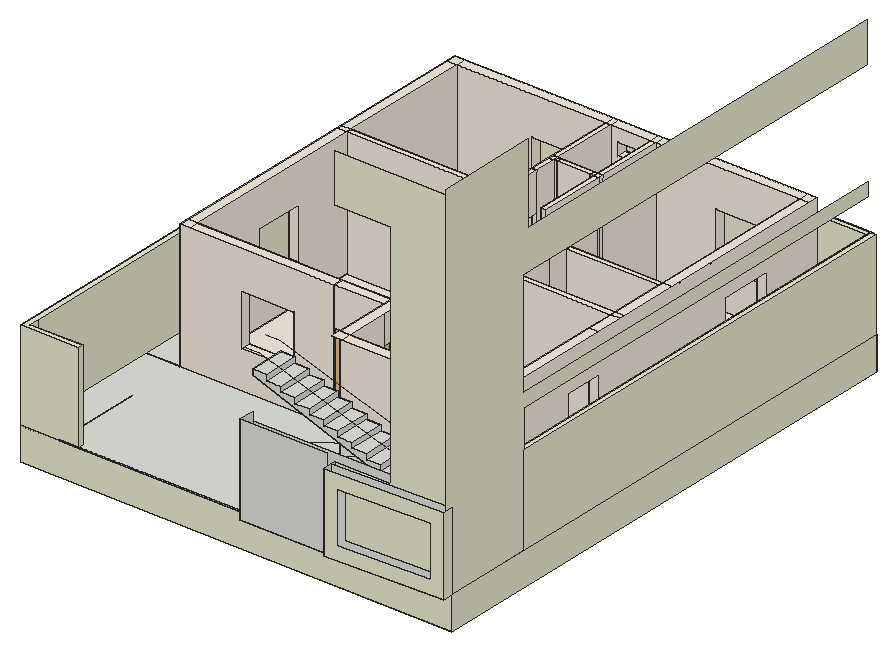
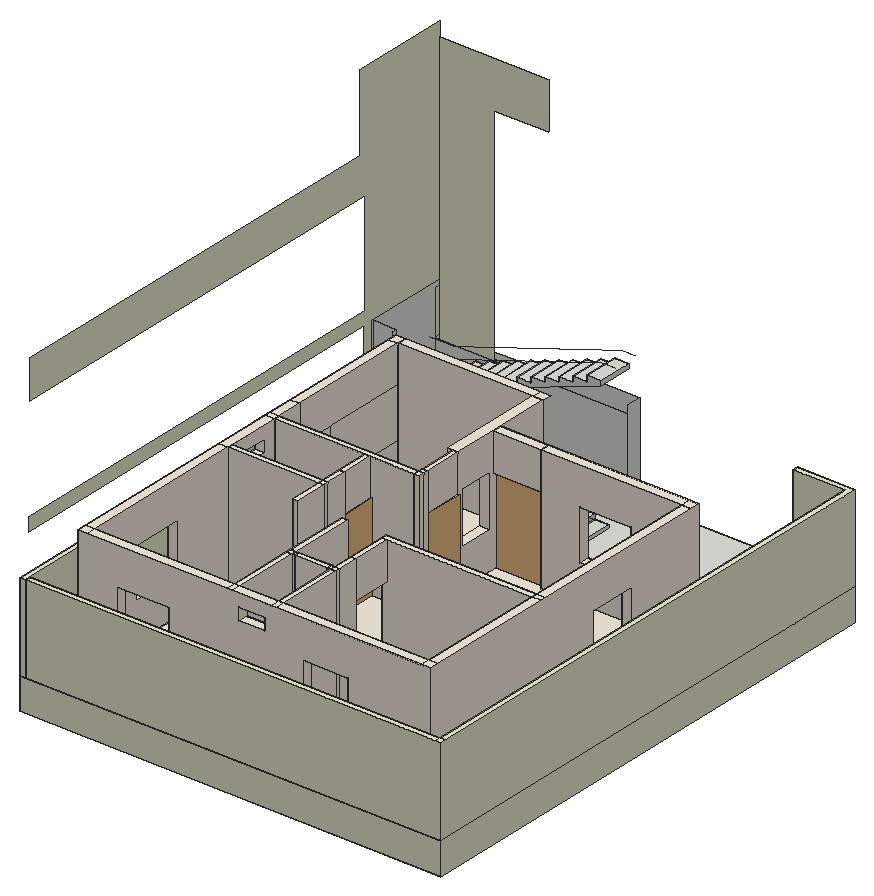
# SketchUp Ruby script. Lengths in inches.
U = 1.inch
M = Sketchup.active_model
def pt(a) = Geom::Point3d.new(a.map { |v| v * U })
def face(e, loops, mat)
  f = e.add_face(loops[0].map { |a| pt(a) })
  loops[1..].each { |l| e.add_face(l.map { |a| pt(a) }).erase! }
  f.material = f.back_material = mat if mat
  f
end
# faces: each face lists its corners as indices into pts; further lists are holes
def faces(e, pts, list, mat = nil) = list.each { |f| face(e, (f[0].is_a?(Array) ? f : [f]).map { |l| l.map { |i| pts[i] } }, mat) }
# xy, xz, yz: faces in a plane at the given z, y or x. An outline is a flat list of corners, or four numbers for a rectangle; further outlines are holes
def ring(l) = l.size == 4 ? [[l[0], l[1]], [l[2], l[1]], [l[2], l[3]], [l[0], l[3]]] : l.each_slice(2).to_a
def flat(e, list, mat, &to3) = list.each { |f| face(e, (f[0].is_a?(Array) ? f : [f]).map { |l| ring(l).map { |u, v| to3.(u, v) } }, mat) }
def xy(e, z, list, mat = nil) = flat(e, list, mat) { |x, y| [x, y, z] }
def xz(e, y, list, mat = nil) = flat(e, list, mat) { |x, z| [x, y, z] }
def yz(e, x, list, mat = nil) = flat(e, list, mat) { |y, z| [x, y, z] }
def lines(e, pts, list) = list.each { |a, b| e.add_line(pt(pts[a]), pt(pts[b])) }
# prism: a flat outline (further loops are holes) pulled along v
def prism(e, loops, v, mat = nil)
  f = face(e, loops, mat); d = Geom::Vector3d.new(v.map { |x| x * U })
  f.pushpull(f.normal.samedirection?(d) ? d.length : -d.length)
end
def box(e, o, s, mat = nil) = prism(e, [[o, [o[0] + s[0], o[1], o[2]], [o[0] + s[0], o[1] + s[1], o[2]], [o[0], o[1] + s[1], o[2]]]], [0, 0, s[2]], mat)
def at(x, y, z, deg = 0) = Geom::Transformation.translation(pt([x, y, z])) * Geom::Transformation.rotation(ORIGIN, Z_AXIS, deg.degrees)
def axes(o, x, y, z) = Geom::Transformation.new([*x, 0, *y, 0, *z, 0, *pt(o).to_a, 1])
def part(name) = M.definitions.add(name)
# library, detail: a bought-in or finely detailed component or shape, given as its bounding box
def library(name, o, s) = part(name).tap { |d| box(d.entities, o, s) }
def detail(e, o, s) = box(e.add_group.entities, o, s)
def put(e, d, t, mat = nil) = e.add_instance(d, t).tap { |i| i.material = mat if mat }
def group(e, t, mat = nil) = e.add_group.tap { |g| g.transformation = t; g.material = mat if mat }.entities
root = M.entities
M.materials.add("0037 AP 8028 PEACH ORGANZA").color = [246, 236, 223]
M.materials.add("0746 AP 7715 LUMINOUS").color = [235, 235, 209]
c1 = library("Group\#12",[0,0,0],[6.9375,42,86.5])
c2 = part("Group19\#2")
p = [[1706.5625,247.76,0],[1706.5625,271.76,0],[1706.5625,427.76,65],[1706.5625,431.76,65],[1720.5625,431.76,65],[1720.5625,427.76,65],
  [1720.5625,283.76,125],[1720.5625,271.76,125],[1686.5625,247.76,0],[1686.5625,271.76,0],[1686.5625,427.76,65],[1686.5625,451.76,65],
  [1740.5625,451.76,65],[1740.5625,427.76,65],[1740.5625,283.76,125],[1740.5625,271.76,125]]
lines(c2.entities,p,[[0,1],[1,2],[2,3],[3,4],[4,5],[5,6],[6,7],[8,9],[9,10],[10,11],[11,12],[12,13],
  [13,14],[14,15]])
c3 = part("Group18\#1")
xy(c3.entities,-3.9375,[[1682.5625,269.14,1710.5625,281.14],[1682.5625,281.14,1710.5625,281.93]])
xy(c3.entities,0.45,[[1682.5625,269.14,1710.5625,281.14]])
xy(c3.entities,6.01,[[1682.5625,281.14,1710.5625,293.14]])
xy(c3.entities,11.58,[[1682.5625,293.14,1710.5625,305.14]])
xy(c3.entities,17.14,[[1682.5625,305.14,1710.5625,317.14]])
xy(c3.entities,22.71,[[1682.5625,317.14,1710.5625,329.14]])
xy(c3.entities,28.27,[[1682.5625,329.14,1710.5625,341.14]])
xy(c3.entities,33.84,[[1682.5625,341.14,1710.5625,353.14]])
xy(c3.entities,39.4,[[1682.5625,353.14,1710.5625,365.14]])
xy(c3.entities,44.97,[[1682.5625,365.14,1710.5625,377.14]])
xy(c3.entities,50.53,[[1682.5625,377.14,1710.5625,389.14]])
xy(c3.entities,56.1,[[1682.5625,389.14,1710.5625,401.14]])
xy(c3.entities,61.66,[[1682.5625,401.14,1710.5625,413.14]])
xy(c3.entities,67.23,[[1682.5625,413.14,1710.5625,425.14]])
xy(c3.entities,68.41,[[1716.5625,412.36,1744.5625,453.14],[1710.5625,425.14,1710.5625,437.93,1682.5625,437.93,1682.5625,453.14,1716.5625,453.14,1716.5625,425.14]])
xy(c3.entities,72.8,[[1716.5625,413.14,1744.5625,453.14],[1682.5625,425.14,1716.5625,453.14]])
xy(c3.entities,78.36,[[1716.5625,401.14,1744.5625,413.14]])
xy(c3.entities,83.93,[[1716.5625,389.14,1744.5625,401.14]])
xy(c3.entities,89.49,[[1716.5625,377.14,1744.5625,389.14]])
xy(c3.entities,95.06,[[1716.5625,365.14,1744.5625,377.14]])
xy(c3.entities,100.62,[[1716.5625,353.14,1744.5625,365.14]])
xy(c3.entities,106.1875,[[1716.5625,341.14,1744.5625,353.14]])
xy(c3.entities,111.75,[[1716.5625,329.14,1744.5625,341.14]])
xy(c3.entities,117.32,[[1716.5625,317.14,1744.5625,329.14]])
xy(c3.entities,122.88,[[1716.5625,305.14,1744.5625,317.14]])
xy(c3.entities,128.45,[[1716.5625,293.14,1744.5625,305.14]])
xy(c3.entities,134.68,[[1716.5625,281.14,1744.5625,293.14]])
xz(c3.entities,269.14,[[1682.5625,-3.9375,1710.5625,0.45]])
xz(c3.entities,281.14,[[1682.5625,-3.9375,1710.5625,0.45],[1682.5625,0.45,1710.5625,6.01],[1716.5625,129.27,1744.5625,134.68]])
xz(c3.entities,293.14,[[1682.5625,6.01,1710.5625,11.58],[1716.5625,128.45,1744.5625,134.68]])
xz(c3.entities,305.14,[[1682.5625,11.58,1710.5625,17.14],[1716.5625,122.88,1744.5625,128.45]])
xz(c3.entities,317.14,[[1682.5625,17.14,1710.5625,22.71],[1716.5625,117.32,1744.5625,122.88]])
xz(c3.entities,329.14,[[1682.5625,22.71,1710.5625,28.27],[1716.5625,111.75,1744.5625,117.32]])
xz(c3.entities,341.14,[[1682.5625,28.27,1710.5625,33.84],[1716.5625,106.1875,1744.5625,111.75]])
xz(c3.entities,353.14,[[1682.5625,33.84,1710.5625,39.4],[1716.5625,100.62,1744.5625,106.1875]])
xz(c3.entities,365.14,[[1682.5625,39.4,1710.5625,44.97],[1716.5625,95.06,1744.5625,100.62]])
xz(c3.entities,377.14,[[1682.5625,44.97,1710.5625,50.53],[1716.5625,89.49,1744.5625,95.06]])
xz(c3.entities,389.14,[[1682.5625,50.53,1710.5625,56.1],[1716.5625,83.93,1744.5625,89.49]])
xz(c3.entities,401.14,[[1682.5625,56.1,1710.5625,61.66],[1716.5625,78.36,1744.5625,83.93]])
xz(c3.entities,413.14,[[1682.5625,61.66,1710.5625,67.23],[1716.5625,72.8,1744.5625,78.36]])
xz(c3.entities,425.14,[[1682.5625,67.23,1710.5625,72.8],[1710.5625,68.41,1716.5625,72.8]])
xz(c3.entities,453.14,[[1682.5625,68.41,1716.5625,72.8],[1716.5625,68.41,1744.5625,72.8]])
yz(c3.entities,1682.5625,[[269.14,-3.9375,281.14,0.45],[281.14,-3.9375,281.14,6.01,293.14,6.01,293.14,11.58,305.14,11.58,305.14,17.14,317.14,17.14,317.14,22.71,329.14,22.71,329.14,28.27,341.14,28.27,341.14,33.84,353.14,33.84,353.14,39.4,365.14,39.4,365.14,44.97,377.14,44.97,377.14,50.53,389.14,50.53,389.14,56.1,401.14,56.1,401.14,61.66,413.14,61.66,413.14,67.23,425.14,67.23,425.14,72.8,453.14,72.8,453.14,68.41,437.93,68.41,281.93,-3.9375]])
yz(c3.entities,1710.5625,[[269.14,-3.9375,281.14,0.45],[281.14,-3.9375,281.93,-3.9375,437.93,68.41,425.14,68.41,425.14,67.23,413.14,67.23,413.14,61.66,401.14,61.66,401.14,56.1,389.14,56.1,389.14,50.53,377.14,50.53,377.14,44.97,365.14,44.97,365.14,39.4,353.14,39.4,353.14,33.84,341.14,33.84,341.14,28.27,329.14,28.27,329.14,22.71,317.14,22.71,317.14,17.14,305.14,17.14,305.14,11.58,293.14,11.58,293.14,6.01,281.14,6.01]])
yz(c3.entities,1716.5625,[[412.36,68.41,281.42,129.14,281.14,129.27,281.14,134.68,293.14,134.68,293.14,128.45,305.14,128.45,305.14,122.88,317.14,122.88,317.14,117.32,329.14,117.32,329.14,111.75,341.14,111.75,341.14,106.1875,353.14,106.1875,353.14,100.62,365.14,100.62,365.14,95.06,377.14,95.06,377.14,89.49,389.14,89.49,389.14,83.93,401.14,83.93,401.14,78.36,413.14,78.36,413.14,72.8,425.14,72.8,425.14,68.41],[425.14,68.41,453.14,72.8]])
yz(c3.entities,1744.5625,[[412.36,68.41,453.14,68.41,453.14,72.8,413.14,72.8,413.14,78.36,401.14,78.36,401.14,83.93,389.14,83.93,389.14,89.49,377.14,89.49,377.14,95.06,365.14,95.06,365.14,100.62,353.14,100.62,353.14,106.1875,341.14,106.1875,341.14,111.75,329.14,111.75,329.14,117.32,317.14,117.32,317.14,122.88,305.14,122.88,305.14,128.45,293.14,128.45,293.14,134.68,281.14,134.68,281.14,129.27]])
p = [[1682.5625,281.93,-3.9375],[1682.5625,437.93,68.41],[1710.5625,437.93,68.41],[1710.5625,281.93,-3.9375],[1744.5625,412.36,68.41],[1744.5625,281.14,129.27],
  [1716.5625,281.42,129.14],[1716.5625,412.36,68.41],[1716.5625,281.14,129.27]]
faces(c3.entities,p,[[0,1,2,3],[4,5,6,7],[8,6,5]])
put(c3.entities,c2,at(0,0,24))
xy(root,-0.68,[[2448.97,99.37,2448.64,108.36,2554.91,112.36,2555.24,103.37],[2370.2,103.36,2370.2,112.52,2550.375,112.52,2550.375,112.36,2448.64,112.36,2448.64,103.36],[2448.64,108.36,2448.64,112.36,2554.91,112.36],[2550.375,112.36,2554.91,112.52],[2370.2,112.52,2550.375,117.53],
  [2550.375,112.52,2554.91,191.07],[2550.375,191.07,2554.91,194.04],[2463.86,337.26,2499.86,337.34,2499.86,337.47,2463.86,337.39]])
xz(root,103.36,[[2370.2,-0.68,2448.64,-0.68,2448.64,69.55,2448.6,69.55,2448.6,80.8,2370.2,80.8]])
xz(root,112.36,[[2448.64,-0.68,2554.91,-0.68,2554.91,69.55,2549.9,69.55,2549.9,322.5,2448.6,322.5,2448.6,278.5,2499.54,278.5,2499.54,69.55,2448.64,69.55]],"0746 AP 7715 LUMINOUS")
xz(root,117.53,[[2370.2,-0.68,2370.2,73.55,2549.9,73.55,2549.9,115.5,2550.375,115.5,2550.375,-0.68]])
xz(root,190.04,[[2528.375,-0.68,2550.375,120]])
yz(root,2370.2,[[103.36,-0.68,103.36,80.8,117.37,80.8,117.37,73.55,117.53,73.55,117.53,-0.68]])
yz(root,2448.64,[[103.36,-0.68,108.36,69.55],[108.36,-0.68,112.36,69.55]])
yz(root,2528.375,[[190.04,-0.68,194.04,120]])
yz(root,2550.375,[[117.53,-0.68,117.53,115.5,112.36,115.5,112.36,120,190.04,120,190.04,-0.68],[190.04,-0.68,191.07,120]])
yz(root,2554.91,[[112.36,-0.68,194.04,-0.68,194.04,115.5,584.4,115.5,584.4,127.5,192.78,127.5,192.78,223.5,583.09,223.5,583.09,259.5,198.89,259.5,198.89,331.5,105.36,331.5,105.36,69.55,112.36,69.55]],"0746 AP 7715 LUMINOUS")
p = [[2448.64,108.36,69.55],[2448.64,108.36,-0.68],[2448.97,99.37,-0.68],[2448.97,99.37,69.55],[2555.24,103.37,69.55],[2555.24,103.37,-0.68],
  [2543.25,102.92,11.32],[2460.97,99.82,11.32],[2460.97,99.82,57.55],[2543.25,102.92,57.55],[2554.91,112.36,-0.68],[2554.91,112.36,69.55],
  [2499.54,110.28,69.55],[2549.9,112.18,69.55],[2460.625,108.82,11.32],[2542.91,111.91,11.32],[2542.91,111.91,57.55],[2499.54,110.28,57.55],
  [2460.625,108.82,57.55]]
faces(root,p,[[0,1,2,3],[[0,12,13,11,10,1],[14,15,16,17,18]]])
faces(root,p,[[[4,3,2,5],[6,7,8,9]],[10,11,4,5]],"0746 AP 7715 LUMINOUS")
g1 = group(root,at(2163.39,579.02,-0.68),"0746 AP 7715 LUMINOUS")
xy(g1,0,[[0,-466.5,5.01,-461.49],[5.01,-466.5,53.01,-461.49],[0,-461.49,5.01,-452.29],[0,-452.29,5.01,9.73],[386.98,-384.97,391.99,14.74],
  [0,9.73,5.01,14.74],[5.01,9.73,386.98,14.74]])
xy(g1,81.48,[[0,-466.5,53.01,-466.5,53.01,-461.49,5.01,-461.49,5.01,9.73,0,9.73],[386.98,-384.97,391.99,14.74],[0,9.73,5.01,14.74],[5.01,9.73,386.98,14.74]])
xz(g1,-466.5,[[0,0,53.01,81.48]])
xz(g1,-461.49,[[5.01,0,53.01,81.48]])
xz(g1,-384.97,[[386.98,0,391.99,81.48]])
xz(g1,9.73,[[5.01,0,386.98,81.48]])
xz(g1,14.74,[[0,0,386.98,81.48],[386.98,0,391.99,81.48]])
yz(g1,0,[[-466.5,0,14.74,81.48]])
yz(g1,5.01,[[-461.49,0,-452.29,81.48],[-452.29,0,9.73,81.48]])
yz(g1,53.01,[[-466.5,0,-461.49,81.48]])
yz(g1,386.98,[[-384.97,0,9.73,81.48],[9.73,0,14.74,81.48]])
yz(g1,391.99,[[-384.97,0,14.74,81.48]])
g2 = group(root,at(2168.4,553.29,-0.68))
xy(g2,0,[[-5.01,-440.77,-5.01,40.47,386.98,40.47,386.98,-440.77,381.97,-440.77,381.97,35.34,0,35.34,0,-435.76,30.99,-435.76,30.99,-440.77],[30.99,-440.77,381.97,-359.24],[0,-435.76,0,-304.77,215.96,-304.77,215.96,-359.24,30.99,-359.24,30.99,-435.76],[359.97,-359.24,381.97,7.26],[0,-304.77,30.99,0],
  [0,0,30.99,7.26],[0,7.26,30.99,35.34],[30.99,7.26,359.97,35.34],[359.97,7.26,381.97,35.34]])
xy(g2,0.97,[[30.99,-440.77,381.97,-440.77,381.97,-359.24,215.96,-359.24,215.96,-304.77,0,-304.77,0,-435.76,30.99,-435.76],[359.97,-359.24,381.97,7.26],[0,-304.77,30.99,0],[0,0,30.99,7.26],[0,7.26,30.99,35.34],
  [30.99,7.26,359.97,35.34],[359.97,7.26,381.97,35.34]])
xz(g2,-440.77,[[30.99,0,381.97,0.97]])
xz(g2,-435.76,[[0,0,30.99,0.97]])
xz(g2,-359.24,[[215.96,0,359.97,0.97]])
xz(g2,-304.77,[[0,0,30.99,0.97],[30.99,0,215.96,0.97]])
xz(g2,0,[[0,0,30.99,0.97]])
xz(g2,7.26,[[0,0,30.99,0.97],[30.99,0,359.97,0.97],[359.97,0,381.97,0.97]])
xz(g2,35.34,[[0,0,30.99,0.97],[30.99,0,359.97,0.97],[359.97,0,381.97,0.97]])
yz(g2,0,[[-435.76,0,-304.77,0.97],[-304.77,0,0,0.97],[0,0,7.26,0.97],[7.26,0,35.34,0.97]])
yz(g2,30.99,[[-440.77,0,-435.76,0.97],[-435.76,0,-359.24,0.97],[-304.77,0,0,0.97],[0,0,7.26,0.97],[7.26,0,35.34,0.97]])
yz(g2,215.96,[[-359.24,0,-304.77,0.97]])
yz(g2,359.97,[[-359.24,0,7.26,0.97],[7.26,0,35.34,0.97]])
yz(g2,381.97,[[-440.77,0,-359.24,0.97],[-359.24,0,7.26,0.97],[7.26,0,35.34,0.97]])
g3 = group(root,at(2163.39,112.52,-30.68),"0746 AP 7715 LUMINOUS")
box(g3,[0,0,0],[392,481.24,30])
put(root,c1,axes([2384.37,249.12,-0.68],[0,0.7279,0],[-1.06713,0,0],[0,0,0.94197]))
g4 = group(root,at(2199.39,551.55,-0.68),"0037 AP 8028 PEACH ORGANZA")
xy(g4,0,[[184.97,-361.51,194,-352.52],[194,-361.51,319.99,-352.52],[319.99,-361.51,328.98,-352.52],[184.97,-352.52,194,-303.04],[194,-352.52,319.99,-303.04],
  [319.99,-352.52,328.98,-303.04],[0,-303.04,8.99,-294.03],[8.99,-303.04,140.15,-294.03],[184.97,-303.04,194,-253.68],[319.99,-303.04,328.98,-238.48],
  [0,-294.03,8.99,-294],[0,-294,8.99,-125],[319.99,-238.48,328.98,-214.09],[184.97,-218.02,189.98,-214.09],[184.97,-214.09,189.98,-209.03],
  [189.98,-214.09,319.99,-209.03],[319.99,-214.09,328.98,-209.03],[319.99,-209.03,328.98,-155.01],[230.99,-179.02,236,-160.01],[230.99,-160.01,236,-155.01],
  [236,-160.01,319.99,-155.01],[230.99,-155.01,236,-125],[319.99,-155.01,328.98,0],[0,-125,8.99,-120.03],[8.99,-125,148.97,-120.03],
  [184.97,-125,189.98,-65.02],[0,-120.03,8.99,0],[144,-84.03,148.97,-65.02],[144,-65.02,148.97,-60.02],[148.97,-65.02,151.97,-60.02],
  [181.98,-65.02,184.97,-60.02],[184.97,-65.02,189.98,-60.02],[144,-60.02,148.97,0],[184.97,-60.02,189.98,0],[0,0,8.99,8.99],
  [8.99,0,144,8.99],[144,0,148.97,8.99],[148.97,0,184.97,8.99],[184.97,0,189.98,8.99],[189.98,0,319.99,8.99],
  [319.99,0,328.98,8.99]])
xy(g4,34.92,[[319.99,-352.52,328.98,-274.28],[55.86,-303.04,103.86,-294.03],[319.99,-274.28,328.98,-238.48],[0,-225,8.99,-179.55],[319.99,-96,328.98,-48],
  [77.49,0,118.65,8.99],[244.5,0,291.95,8.99]])
xy(g4,35.49,[[184.97,-290.84,194,-258.52]])
xy(g4,81.32,[[0,-225,8.99,-179.55]])
xy(g4,81.38,[[77.49,0,118.65,8.99]])
xy(g4,81.48,[[55.86,-303.04,103.86,-294.03],[140.15,-303.04,184.97,-294.03],[319.99,-274.28,328.98,-238.48],[184.97,-253.68,189.49,-218.02],[230.99,-209.03,236.12,-179.02],
  [144,-120.03,148.97,-84.03],[319.99,-96,328.98,-48],[151.97,-65.02,181.98,-60.02],[244.5,0,291.95,8.99]])
xy(g4,83.3,[[184.97,-290.84,194,-258.52]])
xy(g4,93.12,[[319.99,-197.03,328.98,-172.01],[154.97,0,178.97,8.99]])
xy(g4,104.76,[[319.99,-197.03,328.98,-172.01],[154.97,0,178.97,8.99]])
xy(g4,116.4,[[184.97,-361.51,194,-352.52],[194,-361.51,319.99,-352.52],[319.99,-361.51,328.98,-352.52],[184.97,-352.52,194,-253.68],[319.99,-352.52,328.98,-238.48],
  [0,-303.04,8.99,-294.03],[8.99,-303.04,140.15,-294.03],[140.15,-303.04,184.97,-294.03],[0,-294.03,8.99,-294],[0,-294,8.99,-125],
  [184.97,-253.68,189.49,-218.02],[319.99,-238.48,328.98,-214.09],[184.97,-218.02,189.98,-214.09],[184.97,-214.09,189.98,-209.03],[189.98,-214.09,319.99,-209.03],
  [319.99,-214.09,328.98,-209.03],[230.99,-209.03,236.12,-179.02],[319.99,-209.03,328.98,-155.01],[230.99,-179.02,236,-160.01],[230.99,-160.01,236,-155.01],
  [236,-160.01,319.99,-155.01],[230.99,-155.01,236,-125],[319.99,-155.01,328.98,0],[0,-125,8.99,-120.03],[8.99,-125,148.97,-120.03],
  [184.97,-125,189.98,-65.02],[0,-120.03,8.99,0],[144,-120.03,148.97,-84.03],[144,-84.03,148.97,-65.02],[144,-65.02,148.97,-60.02],
  [148.97,-65.02,151.97,-60.02],[151.97,-65.02,181.98,-60.02],[181.98,-65.02,184.97,-60.02],[184.97,-65.02,189.98,-60.02],[144,-60.02,148.97,0],
  [184.97,-60.02,189.98,0],[0,0,8.99,8.99],[8.99,0,144,8.99],[144,0,148.97,8.99],[148.97,0,184.97,8.99],
  [184.97,0,189.98,8.99],[189.98,0,319.99,8.99],[319.99,0,328.98,8.99]])
xz(g4,-361.51,[[319.99,0,328.98,116.4]])
xz(g4,-352.52,[[184.97,0,319.99,116.4],[319.99,0,328.98,34.92]])
xz(g4,-303.04,[[[0,0,140.15,116.4],[55.86,34.92,103.86,81.48]],[140.15,81.48,184.97,116.4]],"0037 AP 8028 PEACH ORGANZA")
xz(g4,-294.03,[[[8.99,0,140.15,116.4],[55.86,34.92,103.86,81.48]],[140.15,81.48,184.97,116.4]])
xz(g4,-290.84,[[184.97,35.49,194,83.3]])
xz(g4,-274.28,[[319.99,34.92,328.98,81.48]])
xz(g4,-258.52,[[184.97,35.49,194,83.3]])
xz(g4,-253.68,[[184.97,0,184.97,81.48,189.49,81.48,189.49,116.4,194,116.4,194,0],[184.97,81.48,189.49,116.4]])
xz(g4,-238.48,[[319.99,0,328.98,34.92],[319.99,34.92,328.98,81.48]])
xz(g4,-225,[[0,34.92,8.99,81.32]])
xz(g4,-218.02,[[184.97,0,189.98,0,189.98,116.4,189.49,116.4,189.49,81.48,184.97,81.48],[184.97,81.48,189.49,116.4]])
xz(g4,-214.09,[[184.97,0,189.98,116.4],[189.98,0,319.99,116.4]])
xz(g4,-209.03,[[184.97,0,189.98,116.4],[189.98,0,189.98,116.4,230.99,116.4,230.99,81.48,236.12,81.48,236.12,116.4,319.99,116.4,319.99,0],[230.99,81.48,236.12,116.4]])
xz(g4,-197.03,[[319.99,93.12,328.98,104.76]])
xz(g4,-179.55,[[0,34.92,8.99,81.32]])
xz(g4,-179.02,[[230.99,0,236,81.48],[230.99,81.48,236,116.4],[236,81.48,236.12,116.4]])
xz(g4,-172.01,[[319.99,93.12,328.98,104.76]])
xz(g4,-160.01,[[230.99,0,236,116.4],[236,0,319.99,116.4]])
xz(g4,-155.01,[[230.99,0,236,116.4],[236,0,319.99,116.4]])
xz(g4,-125,[[8.99,0,148.97,116.4],[184.97,0,189.98,116.4],[230.99,0,236,116.4]])
xz(g4,-120.03,[[8.99,0,8.99,116.4,144,116.4,144,81.48,148.97,81.48,148.97,0],[144,81.48,148.97,116.4]])
xz(g4,-96,[[319.99,34.92,328.98,81.48]])
xz(g4,-84.03,[[144,0,148.97,81.48],[144,81.48,148.97,116.4]])
xz(g4,-65.02,[[144,0,148.97,116.4],[148.97,0,151.97,116.4],[181.98,0,184.97,116.4],[184.97,0,189.98,116.4],[151.97,81.48,181.98,116.4]])
xz(g4,-60.02,[[144,0,148.97,116.4],[148.97,0,151.97,116.4],[181.98,0,184.97,116.4],[184.97,0,189.98,116.4],[151.97,81.48,181.98,116.4]])
xz(g4,-48,[[319.99,34.92,328.98,81.48]])
xz(g4,0,[[[8.99,0,144,116.4],[77.49,34.92,118.65,81.38]],[144,0,148.97,116.4],[[148.97,0,184.97,116.4],[154.97,93.12,178.97,104.76]],[184.97,0,189.98,116.4],[[189.98,0,319.99,116.4],[244.5,34.92,291.95,81.48]]])
xz(g4,8.99,[[[0,0,328.98,116.4],[244.5,34.92,291.95,81.48],[77.49,34.92,118.65,81.38],[154.97,93.12,178.97,104.76]]])
yz(g4,0,[[[-303.04,0,8.99,116.4],[-225,34.92,-179.55,81.32]]],"0037 AP 8028 PEACH ORGANZA")
yz(g4,8.99,[[-294.03,0,-294,116.4],[[-294,0,-125,116.4],[-225,34.92,-179.55,81.32]],[-125,0,-120.03,116.4],[-120.03,0,0,116.4]])
yz(g4,55.86,[[-303.04,34.92,-294.03,81.48]])
yz(g4,77.49,[[0,34.92,8.99,81.38]])
yz(g4,103.86,[[-303.04,34.92,-294.03,81.48]])
yz(g4,118.65,[[0,34.92,8.99,81.38]])
yz(g4,140.15,[[-303.04,0,-294.03,81.48],[-303.04,81.48,-294.03,116.4]])
yz(g4,144,[[-84.03,0,-65.02,116.4],[-65.02,0,-60.02,116.4],[-60.02,0,0,116.4],[-120.03,81.48,-84.03,116.4]])
yz(g4,148.97,[[-125,0,-120.03,116.4],[-84.03,0,-65.02,116.4],[-65.02,0,-60.02,116.4],[-60.02,0,0,116.4],[-120.03,81.48,-84.03,116.4]])
yz(g4,151.97,[[-65.02,0,-60.02,81.48],[-65.02,81.48,-60.02,116.4]])
yz(g4,154.97,[[0,93.12,8.99,104.76]])
yz(g4,178.97,[[0,93.12,8.99,104.76]])
yz(g4,181.98,[[-65.02,0,-60.02,81.48],[-65.02,81.48,-60.02,116.4]])
yz(g4,184.97,[[[-352.52,0,-352.52,116.4,-303.04,116.4,-303.04,81.48,-294.03,81.48,-294.03,116.4,-253.68,116.4,-253.68,0],[-290.84,35.49,-258.52,83.3]],[-218.02,0,-214.09,116.4],[-214.09,0,-209.03,116.4],[-125,0,-65.02,116.4],[-65.02,0,-60.02,116.4],
  [-60.02,0,0,116.4],[-303.04,81.48,-294.03,116.4],[-253.68,81.48,-218.02,116.4]])
yz(g4,189.49,[[-253.68,81.48,-218.02,116.4]])
yz(g4,189.98,[[-218.02,0,-214.09,116.4],[-214.09,0,-209.03,116.4],[-125,0,-65.02,116.4],[-65.02,0,-60.02,116.4],[-60.02,0,0,116.4]])
yz(g4,230.99,[[-179.02,0,-160.01,116.4],[-160.01,0,-155.01,116.4],[-155.01,0,-125,116.4],[-209.03,81.48,-179.02,116.4]])
yz(g4,236,[[-179.02,0,-160.01,116.4],[-160.01,0,-155.01,116.4],[-155.01,0,-125,116.4]])
yz(g4,236.12,[[-209.03,81.48,-179.02,116.4]])
yz(g4,244.5,[[0,34.92,8.99,81.48]])
yz(g4,291.95,[[0,34.92,8.99,81.48]])
yz(g4,319.99,[[-361.51,0,-352.52,116.4],[-352.52,0,-280.02,34.92],[-280.02,0,-238.48,34.92],[-238.48,0,-214.09,116.4],[-214.09,0,-209.03,116.4],
  [[-209.03,0,-160.01,116.4],[-197.03,93.12,-172.01,104.76]],[-160.01,0,-155.01,116.4],[[-155.01,0,0,116.4],[-96,34.92,-48,81.48]],[-352.52,34.92,-274.28,81.48],[-352.52,81.48,-238.48,116.4]])
yz(g4,328.98,[[[-361.51,0,-352.52,0,-352.52,34.92,-274.28,34.92,-274.28,81.48,-238.48,81.48,-238.48,0,8.99,0,8.99,116.4,-361.51,116.4],[-96,34.92,-48,81.48],[-197.03,93.12,-172.01,104.76]],[-352.52,0,-238.48,34.92]])
# 3 loose lines left out
g5 = group(g4,at(8.99,-303.04,0))
prism(g5,[[[311,0,0],[185.01,0,0],[185.01,49.36,0],[175.98,49.36,0],[175.98,0,0],[131.16,0,0],[131.16,9.01,0],[0,9.01,0],[0,9.03,0],[0,178.04,0],[139.98,178.04,0],[139.98,183,0],[0,183,0],[0,303.04,0],[135.02,303.04,0],[135.02,243.02,0],[135.02,238.01,0],[135.02,219,0],[139.98,219,0],[139.98,238.01,0],[142.98,238.01,0],[142.98,243.02,0],[139.98,243.02,0],[139.98,303.04,0],[175.98,303.04,0],[175.98,243.02,0],[172.99,243.02,0],[172.99,238.01,0],[175.98,238.01,0],[175.98,178.04,0],[180.99,178.04,0],[180.99,238.01,0],[180.99,243.02,0],[180.99,303.04,0],[311,303.04,0],[311,148.03,0],[227.01,148.03,0],[227.01,178.04,0],[222,178.04,0],[222,148.03,0],[222,143.02,0],[222,124.01,0],[227.01,124.01,0],[227.01,143.02,0],[311,143.02,0],[311,94.01,0],[180.99,94.01,0],[175.98,94.01,0],[175.98,88.95,0],[175.98,85.02,0],[180.99,85.02,0],[180.99,88.95,0],[311,88.95,0],[311,64.55,0],[311,23.02,0]]],[0,0,0.97])
put(root,c1,axes([2382.07,486.49,-0.68],[0,0.7279,0],[-0.73015,0,0],[0,0,0.94197]))
put(root,c1,axes([2382.94,297.875,-0.68],[0.85622,0,0],[0,0.84902,0],[0,0,0.94197]))
put(root,c1,axes([2428.96,341.86,-0.68],[0.92718,0,0],[0,0.73015,0],[0,0,0.94197]))
put(root,c3,axes([2050.35,2146.65,2.62],[0.0107,-1.16479,0],[1.07101,0.00984,0],[0,0,0.83812]))
